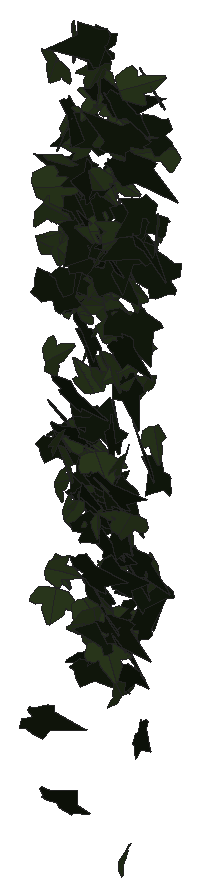
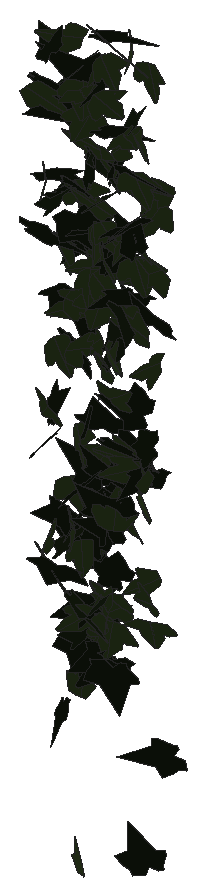
# SketchUp Ruby script. Lengths in inches.
U = 1.inch
M = Sketchup.active_model
def pt(a) = Geom::Point3d.new(a.map { |v| v * U })
def face(e, loops, mat)
  f = e.add_face(loops[0].map { |a| pt(a) })
  loops[1..].each { |l| e.add_face(l.map { |a| pt(a) }).erase! }
  f.material = f.back_material = mat if mat
  f
end
# faces: each face lists its corners as indices into pts; further lists are holes
def faces(e, pts, list, mat = nil) = list.each { |f| face(e, (f[0].is_a?(Array) ? f : [f]).map { |l| l.map { |i| pts[i] } }, mat) }
# xy, xz, yz: faces in a plane at the given z, y or x. An outline is a flat list of corners, or four numbers for a rectangle; further outlines are holes
def ring(l) = l.size == 4 ? [[l[0], l[1]], [l[2], l[1]], [l[2], l[3]], [l[0], l[3]]] : l.each_slice(2).to_a
def flat(e, list, mat, &to3) = list.each { |f| face(e, (f[0].is_a?(Array) ? f : [f]).map { |l| ring(l).map { |u, v| to3.(u, v) } }, mat) }
def xy(e, z, list, mat = nil) = flat(e, list, mat) { |x, y| [x, y, z] }
def xz(e, y, list, mat = nil) = flat(e, list, mat) { |x, z| [x, y, z] }
def yz(e, x, list, mat = nil) = flat(e, list, mat) { |y, z| [x, y, z] }
def lines(e, pts, list) = list.each { |a, b| e.add_line(pt(pts[a]), pt(pts[b])) }
# prism: a flat outline (further loops are holes) pulled along v
def prism(e, loops, v, mat = nil)
  f = face(e, loops, mat); d = Geom::Vector3d.new(v.map { |x| x * U })
  f.pushpull(f.normal.samedirection?(d) ? d.length : -d.length)
end
def box(e, o, s, mat = nil) = prism(e, [[o, [o[0] + s[0], o[1], o[2]], [o[0] + s[0], o[1] + s[1], o[2]], [o[0], o[1] + s[1], o[2]]]], [0, 0, s[2]], mat)
def at(x, y, z, deg = 0) = Geom::Transformation.translation(pt([x, y, z])) * Geom::Transformation.rotation(ORIGIN, Z_AXIS, deg.degrees)
def axes(o, x, y, z) = Geom::Transformation.new([*x, 0, *y, 0, *z, 0, *pt(o).to_a, 1])
def part(name) = M.definitions.add(name)
# library, detail: a bought-in or finely detailed component or shape, given as its bounding box
def library(name, o, s) = part(name).tap { |d| box(d.entities, o, s) }
def detail(e, o, s) = box(e.add_group.entities, o, s)
def put(e, d, t, mat = nil) = e.add_instance(d, t).tap { |i| i.material = mat if mat }
def group(e, t, mat = nil) = e.add_group.tap { |g| g.transformation = t; g.material = mat if mat }.entities
root = M.entities
M.materials.add("1026 AP 7946 SUNNY SIDE UP").color = [254, 231, 186]
M.materials.add("efeu1").color = [18, 25, 13]
M.materials.add("efeu2").color = [43, 57, 29]
c1 = part("ivyleaf_10")
p = [[0,0.5,-0.03],[-0.0625,2.02,-0.43],[-0.19,2.01,-0.46],[-0.54,1.05,-0.29],[-0.52,0.625,-0.18],[-0.83,0.76,-0.28],
  [-1.16,0.64,-0.33],[-1.15,0.33,-0.24],[-0.77,-0.39,0.02],[-0.3,-0.51,0.16],[0.04,-0.48,0.23],[-0.02,2.01,-0.4375],
  [-0.06,2.01,-0.43],[0.04,-0.49,0.23],[0.67,-0.49,0.14],[1.38,0.36,-0.2],[1.375,0.51,-0.24],[0.81,0.65,-0.19],
  [0.62,0.59,-0.15],[0.6,1.09,-0.28],[0.5,1.23,-0.31]]
faces(c1.entities,p,[[0,1,2,3,4,5,6,7,8,9,10],[11,12,0,13,14,15,16,17,18,19,20]],"efeu2")
c2 = part("ivyleaf_9")
p = [[1.54,2.16,1.25],[1.36,2.04,1.19],[-0.21,0.99,0.68],[-0.71,1.11,0.82],[-0.85,0.86,0.67],[-0.8,0.17,0.21],
  [-0.9,-0.01,0.1],[-0.67,-0.16,-0.02],[-0.08,-0.08,-0.05],[-0.03,-0.6,-0.4],[0.65,-0.88,-0.66],[0.83,-0.6,-0.49],
  [1.29,-0.42,-0.43],[1.8125,-0.07,-0.26],[1.21,0.44,0.15]]
faces(c2.entities,p,[[0,1,2,3,4,5,6,7,8,9,10,11,12,13,14]],"efeu1")
put(root,c1,axes([114.66,211.24,255.74],[-0.17007,-0.25209,-0.06808],[0.06713,0.05188,-0.28166],[0.40367,-0.11483,0.01816]),"1026 AP 7946 SUNNY SIDE UP")
put(root,c2,axes([114.43,211.45,264.72],[-0.03264,-0.0088,0.26998],[-0.17282,-0.23845,-0.01861],[0.37443,-0.11082,0.01495]),"1026 AP 7946 SUNNY SIDE UP")
put(root,c1,axes([115.3,211.32,264.08],[-0.30301,-0.12678,0.13717],[-0.15655,-0.09143,-0.23738],[0.244,-0.21609,0.01804]),"1026 AP 7946 SUNNY SIDE UP")
put(root,c1,axes([114.875,211.3,255],[0.39379,0.04754,0.12039],[0.18826,-0.00959,-0.26097],[-0.06127,0.27608,-0.02813]),"1026 AP 7946 SUNNY SIDE UP")
put(root,c1,axes([113.82,211.09,256.41],[0.04108,0.08662,0.235],[0.07694,0.22239,-0.09167],[-0.37514,0.0551,0.00693]),"1026 AP 7946 SUNNY SIDE UP")
put(root,c2,axes([114.28,211.5,263.51],[-0.16249,-0.21094,0.17183],[-0.07271,-0.16337,-0.2416],[0.41773,-0.11049,0.02478]),"1026 AP 7946 SUNNY SIDE UP")
put(root,c2,axes([115.59,211.3,257.2],[0.02088,-0.02394,-0.25705],[0.3777,0.07217,0.00646],[0.11192,-0.23908,0.02615]),"1026 AP 7946 SUNNY SIDE UP")
put(root,c2,axes([115.05,211.33,256.57],[0.04614,0.00383,0.26116],[0.28307,-0.17999,-0.01972],[0.28067,0.18089,-0.02304]),"1026 AP 7946 SUNNY SIDE UP")
put(root,c2,axes([115.49,211.22,265.66],[-0.01709,-0.02402,-0.30405],[0.35249,0.19209,-0.02349],[0.30389,-0.22416,0.01015]),"1026 AP 7946 SUNNY SIDE UP")
put(root,c2,axes([115.65,211.44,263.92],[-0.30341,-0.11682,0.11722],[-0.13955,-0.07389,-0.23227],[0.216,-0.21183,0.0146]),"1026 AP 7946 SUNNY SIDE UP")
put(root,c1,axes([113.54,211.17,264.51],[0.12534,-0.00768,-0.2999],[0.42709,0.11067,0.07427],[0.16492,-0.28076,0.03558]),"1026 AP 7946 SUNNY SIDE UP")
put(root,c1,axes([113.61,211.15,264.12],[-0.1046,-0.20587,-0.24089],[0.18057,0.20479,-0.21931],[0.4539,-0.12891,0.03173]),"1026 AP 7946 SUNNY SIDE UP")
put(root,c2,axes([114.8,211.375,258.32],[0.04947,-0.07557,0.27589],[0.34471,-0.15995,-0.07385],[0.27054,0.21762,0.04365]),"1026 AP 7946 SUNNY SIDE UP")
put(root,c1,axes([114.51,211.43,257.81],[0.22659,-0.07934,0.20756],[0.24435,-0.13141,-0.16821],[0.23805,0.21041,-0.0249]),"1026 AP 7946 SUNNY SIDE UP")
put(root,c2,axes([115.31,211.41,260.83],[-0.18396,-0.02952,-0.27245],[0.41815,-0.01085,-0.12008],[0.0031,-0.28883,0.03065]),"1026 AP 7946 SUNNY SIDE UP")
put(root,c2,axes([114.97,211.49,255.23],[-0.12645,-0.02112,0.26836],[-0.28963,-0.18894,-0.07543],[0.29179,-0.19669,0.04142]),"1026 AP 7946 SUNNY SIDE UP")
put(root,c2,axes([114.96,211.24,263.16],[0.11119,-0.17412,-0.20533],[-0.01889,0.20299,-0.18682],[0.41455,0.05595,0.04656]),"1026 AP 7946 SUNNY SIDE UP")
put(root,c1,axes([114.98,211.4,265.1],[-0.07258,-0.05386,-0.264],[0.34796,-0.14661,-0.01019],[-0.21927,-0.21483,0.07122]),"1026 AP 7946 SUNNY SIDE UP")
put(root,c1,axes([114.59,211.4,264.96],[-0.22027,0.03601,-0.22286],[0.26472,-0.14719,-0.13829],[-0.22147,-0.21176,0.05635]),"1026 AP 7946 SUNNY SIDE UP")
put(root,c2,axes([115.13,211.4,261.6],[0.0724,-0.05469,-0.27668],[0.42883,0.03311,0.04146],[0.0379,-0.27017,0.05943]),"1026 AP 7946 SUNNY SIDE UP")
put(root,c2,axes([114.66,211.5,263.34],[0.09706,-0.13204,0.269],[0.13776,-0.24708,-0.15107],[0.44008,0.10646,-0.01204]),"1026 AP 7946 SUNNY SIDE UP")
put(root,c2,axes([116,211.25,259.24],[0.00962,-0.17645,0.2395],[-0.01877,0.23319,0.18324],[-0.4598,-0.01321,-0.00247]),"1026 AP 7946 SUNNY SIDE UP")
put(root,c1,axes([115.4,211.36,257.95],[-0.33522,-0.14331,0.08976],[-0.09251,-0.06946,-0.26394],[0.24768,-0.21991,0.02291]),"1026 AP 7946 SUNNY SIDE UP")
put(root,c1,axes([113.6,211.36,255.67],[0.38787,0.0925,-0.01096],[-0.00313,-0.02634,-0.27043],[-0.14647,0.24552,-0.02323]),"1026 AP 7946 SUNNY SIDE UP")
put(root,c2,axes([114.35,211.38,256.41],[0.08918,-0.01835,0.26004],[0.30281,-0.16487,-0.05787],[0.25845,0.1995,-0.02193]),"1026 AP 7946 SUNNY SIDE UP")
put(root,c1,axes([114.86,211.39,261.15],[-0.24924,0.15249,-0.16603],[0.15304,-0.13138,-0.22624],[-0.31462,-0.18471,0.02148]),"1026 AP 7946 SUNNY SIDE UP")
put(root,c2,axes([113.28,211.19,253.03],[0.1264,0.03867,-0.24017],[0.12708,0.22714,0.06879],[0.34954,-0.09656,0.06184]),"1026 AP 7946 SUNNY SIDE UP")
put(root,c2,axes([114.92,211.29,255.56],[-0.03216,-0.04064,-0.27817],[0.30762,0.18639,-0.04311],[0.29902,-0.19612,0.01444]),"1026 AP 7946 SUNNY SIDE UP")
put(root,c2,axes([115.7,211.31,255.73],[-0.09753,0.22615,0.16908],[0.07272,-0.15616,0.24065],[0.43212,0.07732,-0.00234]),"1026 AP 7946 SUNNY SIDE UP")
put(root,c1,axes([113.8,211.38,258.8],[-0.21862,0.17295,-0.11784],[0.09605,-0.09868,-0.22881],[-0.31247,-0.15134,0.01212]),"1026 AP 7946 SUNNY SIDE UP")
put(root,c1,axes([114.41,211.35,255.73],[0.29749,0.06497,0.17027],[0.26175,0.01771,-0.20383],[-0.09571,0.25035,-0.0282]),"1026 AP 7946 SUNNY SIDE UP")
put(root,c1,axes([113.69,211.13,260.9],[0.04669,-0.00574,-0.30414],[0.15125,0.28068,0.00598],[0.43892,-0.09611,0.03029]),"1026 AP 7946 SUNNY SIDE UP")
put(root,c2,axes([114.72,211.49,256.97],[0.07288,-0.04471,0.28318],[0.22679,-0.23482,-0.06571],[0.37505,0.15068,-0.01529]),"1026 AP 7946 SUNNY SIDE UP")
put(root,c1,axes([114.55,211.36,255.27],[-0.42453,-0.06949,-0.01035],[0.02571,-0.02499,-0.28587],[0.10728,-0.269,0.02753]),"1026 AP 7946 SUNNY SIDE UP")
put(root,c2,axes([115.36,211.39,265.92],[0.00099,0.0417,0.27274],[-0.41206,0.0545,-0.00789],[-0.0866,-0.25884,0.04066]),"1026 AP 7946 SUNNY SIDE UP")
put(root,c2,axes([114.54,211.4375,257.76],[0.30374,-0.14164,0.10657],[-0.1091,0.08092,0.24617],[-0.2541,-0.20404,0.02169]),"1026 AP 7946 SUNNY SIDE UP")
put(root,c1,axes([113.63,211.5,258.05],[0.08777,-0.1533,-0.2045],[0.15271,-0.17333,0.16575],[-0.36243,-0.11015,0.02031]),"1026 AP 7946 SUNNY SIDE UP")
put(root,c2,axes([114.36,211.44,257.76],[-0.00977,-0.02193,0.26649],[0.28374,-0.18656,-0.01292],[0.29374,0.17948,0.02134]),"1026 AP 7946 SUNNY SIDE UP")
put(root,c2,axes([115.18,211.33,257.51],[0.17287,-0.16507,-0.15645],[-0.15698,0.11428,-0.20301],[0.31472,0.14767,-0.01532]),"1026 AP 7946 SUNNY SIDE UP")
put(root,c1,axes([114.56,211.48,255.8],[-0.13203,0.02969,0.24357],[0.33412,-0.10372,0.09062],[0.16897,0.22828,0.01113]),"1026 AP 7946 SUNNY SIDE UP")
put(root,c2,axes([114.22,211.59,261.51],[0.04531,-0.20769,0.19512],[0.03591,-0.18923,-0.2171],[0.44178,0.03668,-0.00237]),"1026 AP 7946 SUNNY SIDE UP")
put(root,c1,axes([113.72,211.43,259.14],[0.05475,-0.24728,0.00725],[-0.00329,-0.00881,-0.25728],[0.38903,0.03472,-0.00319]),"1026 AP 7946 SUNNY SIDE UP")
put(root,c2,axes([114.27,211.62,261.06],[-0.03174,-0.12777,0.26578],[0.03799,-0.25919,-0.13144],[0.45212,0.01281,0.0297]),"1026 AP 7946 SUNNY SIDE UP")
put(root,c1,axes([114.67,211.39,263.85],[0.20477,-0.05823,-0.22915],[0.35388,-0.01823,0.14076],[-0.07154,-0.25682,0.04038]),"1026 AP 7946 SUNNY SIDE UP")
put(root,c1,axes([113.96,211.41,257.5],[0.32931,-0.17306,-0.04965],[0.08071,-0.01173,0.27878],[-0.27028,-0.21436,0.02275]),"1026 AP 7946 SUNNY SIDE UP")
put(root,c1,axes([114.62,211.4,258.91],[0.33119,0.14616,0.07968],[0.11985,0.02385,-0.26292],[-0.23008,0.22282,-0.02225]),"1026 AP 7946 SUNNY SIDE UP")
put(root,c1,axes([113.68,211.37,267.09],[-0.34648,0.10045,0.1055],[-0.17571,-0.00413,-0.24493],[-0.14042,-0.24271,0.04617]),"1026 AP 7946 SUNNY SIDE UP")
put(root,c2,axes([115.26,211.36,254.75],[0.31164,0.03666,-0.16069],[-0.23369,-0.05154,-0.20705],[-0.09501,0.24702,-0.01781]),"1026 AP 7946 SUNNY SIDE UP")
put(root,c2,axes([113.73,211.51,260.06],[0.2403,-0.11574,0.21856],[0.23253,-0.15472,-0.197],[0.3017,0.21144,-0.02225]),"1026 AP 7946 SUNNY SIDE UP")
put(root,c1,axes([113.52,211.51,256.24],[0.16121,-0.00611,0.21576],[0.3107,-0.07483,-0.10232],[0.10972,0.22088,-0.02726]),"1026 AP 7946 SUNNY SIDE UP")
put(root,c2,axes([113.93,211.6875,265.85],[-0.02854,-0.19514,0.25533],[-0.02292,-0.24858,-0.20329],[0.49685,-0.02267,0.00529]),"1026 AP 7946 SUNNY SIDE UP")
put(root,c2,axes([114.56,211.32,254.6],[-0.00266,-0.10371,-0.2671],[0.01774,0.25845,-0.10531],[0.43787,-0.0111,0.00265]),"1026 AP 7946 SUNNY SIDE UP")
put(root,c1,axes([115.06,211.59,253.98],[-0.08601,-0.20779,-0.16962],[-0.04609,-0.16113,0.22017],[-0.41316,0.06123,0.01075]),"1026 AP 7946 SUNNY SIDE UP")
put(root,c2,axes([114.72,211.47,262.72],[0.13518,-0.1909,0.13804],[-0.02992,0.13773,0.2138],[-0.36649,-0.08165,0.03346]),"1026 AP 7946 SUNNY SIDE UP")
put(root,c1,axes([115.13,211.67,260.94],[-0.0853,-0.03267,0.29358],[0.02072,-0.29018,-0.03337],[0.45084,0.00716,0.05708]),"1026 AP 7946 SUNNY SIDE UP")
put(root,c1,axes([114.13,211.625,265.4],[-0.04069,0.09275,0.24744],[0.02887,-0.23959,0.09617],[0.40305,0.02652,0.01809]),"1026 AP 7946 SUNNY SIDE UP")
put(root,c2,axes([115.42,211.54,264.3125],[-0.38926,0.02006,-0.04618],[0.06741,-0.02532,-0.25506],[-0.03801,-0.25033,0.02061]),"1026 AP 7946 SUNNY SIDE UP")
put(root,c2,axes([114.38,211.31,257.33],[0.053,0.04424,0.26084],[0.37301,0.09229,-0.04866],[-0.15456,0.2379,-0.02798]),"1026 AP 7946 SUNNY SIDE UP")
put(root,c2,axes([114.53,211.41,258.38],[-0.20288,0.10014,0.21062],[0.27908,-0.10187,0.16667],[0.22288,0.21871,-0.01698]),"1026 AP 7946 SUNNY SIDE UP")
put(root,c2,axes([114.48,211.57,256.03],[0.15726,-0.25847,0.02263],[0.0048,-0.02393,-0.2856],[0.40806,0.0999,-0.00536]),"1026 AP 7946 SUNNY SIDE UP")
put(root,c1,axes([113.76,211.5625,265.73],[0.19013,-0.21589,0.08202],[0.04409,-0.07684,-0.25504],[0.35979,0.1235,-0.01209]),"1026 AP 7946 SUNNY SIDE UP")
put(root,c1,axes([115.32,211.59,262.68],[-0.13872,0.07861,0.27248],[0.36566,-0.12742,0.11838],[0.23228,0.24753,-0.02362]),"1026 AP 7946 SUNNY SIDE UP")
put(root,c1,axes([115.17,211.47,259.15],[0.04188,-0.28273,-0.06084],[-0.00235,0.05756,-0.2922],[0.45365,0.0264,0.0041]),"1026 AP 7946 SUNNY SIDE UP")
put(root,c2,axes([114.97,211.57,255.19],[0.22849,-0.21422,0.05526],[0.02806,-0.05407,-0.26652],[0.34657,0.14561,-0.01486]),"1026 AP 7946 SUNNY SIDE UP")
put(root,c2,axes([114.68,211.42,259.44],[-0.32119,-0.00531,0.14945],[0.22806,-0.01912,0.20952],[0.01063,0.24983,0.02068]),"1026 AP 7946 SUNNY SIDE UP")
put(root,c2,axes([114.54,211.62,267.64],[-0.33393,-0.00971,0.16324],[-0.2327,-0.0839,-0.21005],[0.09058,-0.25137,0.06217]),"1026 AP 7946 SUNNY SIDE UP")
put(root,c1,axes([114.43,211.61,260.74],[0.05075,-0.08601,-0.23648],[0.23756,-0.17473,0.0885],[-0.30262,-0.15159,0.02982]),"1026 AP 7946 SUNNY SIDE UP")
put(root,c2,axes([115.51,211.59,263.96],[0.20555,-0.25103,0.03547],[0.01146,-0.0366,-0.29159],[0.39856,0.13051,-0.00991]),"1026 AP 7946 SUNNY SIDE UP")
put(root,c1,axes([115.15,211.67,261.95],[-0.05558,-0.12647,0.22673],[-0.05695,-0.21815,-0.13597],[0.39603,-0.04912,0.01227]),"1026 AP 7946 SUNNY SIDE UP")
put(root,c2,axes([113.78,211.5625,259.05],[0.37981,-0.02151,-0.02187],[0.03629,0.02235,0.24871],[-0.03048,-0.24144,0.02354]),"1026 AP 7946 SUNNY SIDE UP")
put(root,c2,axes([114.18,211.46,264.85],[-0.19437,0.13254,0.19459],[-0.29028,0.07039,-0.17564],[-0.21604,-0.21382,0.06093]),"1026 AP 7946 SUNNY SIDE UP")
put(root,c1,axes([115.58,211.58,260.85],[-0.11909,-0.27542,0.06823],[-0.01917,-0.06694,-0.2946],[0.44559,-0.07649,0.00556]),"1026 AP 7946 SUNNY SIDE UP")
put(root,c2,axes([114.91,211.62,263.47],[-0.10304,-0.2649,-0.05673],[0.02722,0.05089,-0.28078],[0.42408,-0.06763,0.00424]),"1026 AP 7946 SUNNY SIDE UP")
put(root,c1,axes([114.51,211.58,263.62],[-0.27553,-0.13701,0.11319],[-0.11756,-0.08345,-0.22892],[0.25073,-0.1897,0.01705]),"1026 AP 7946 SUNNY SIDE UP")
put(root,c2,axes([115.06,211.51,266.81],[0.22169,-0.22399,-0.11841],[-0.05999,0.10974,-0.27089],[0.39038,0.14407,0.02561]),"1026 AP 7946 SUNNY SIDE UP")
put(root,c1,axes([115.77,211.66,256.74],[-0.10353,0.13953,0.22415],[0.15244,-0.19393,0.15779],[0.37563,0.11716,-0.00225]),"1026 AP 7946 SUNNY SIDE UP")
put(root,c2,axes([114.41,211.68,265.74],[-0.3294,-0.08627,0.13607],[-0.16654,-0.0869,-0.23118],[0.18472,-0.23219,0.03423]),"1026 AP 7946 SUNNY SIDE UP")
put(root,c2,axes([115.13,211.57,263.66],[-0.00973,0.20677,-0.223],[-0.03129,-0.21748,-0.21355],[-0.47099,0.01018,0.01879]),"1026 AP 7946 SUNNY SIDE UP")
put(root,c2,axes([115.71,211.7,264.42],[-0.32129,-0.13757,0.1002],[-0.10281,-0.07748,-0.25282],[0.24493,-0.21298,0.02532]),"1026 AP 7946 SUNNY SIDE UP")
put(root,c1,axes([113.83,211.55,264.87],[-0.36323,-0.04128,0.10677],[-0.14616,-0.06152,-0.2385],[0.09763,-0.2457,0.0402]),"1026 AP 7946 SUNNY SIDE UP")
put(root,c1,axes([115.38,211.36,267.18],[0.12226,0.03109,-0.29225],[0.3264,0.19587,0.08182],[0.30834,-0.21967,0.02927]),"1026 AP 7946 SUNNY SIDE UP")
put(root,c2,axes([114.67,211.34,264.73],[-0.2767,0.21118,-0.08365],[-0.06078,0.07483,0.28305],[0.35122,0.17932,-0.01692]),"1026 AP 7946 SUNNY SIDE UP")
put(root,c2,axes([115.16,211.68,257.05],[0.15116,-0.28344,0.06843],[0.02159,-0.06716,-0.30861],[0.45784,0.09675,-0.00804]),"1026 AP 7946 SUNNY SIDE UP")
put(root,c2,axes([113.53,211.45,261.98],[-0.28326,0.18516,0.18087],[0.22182,-0.10528,0.26447],[0.33298,0.22765,-0.02231]),"1026 AP 7946 SUNNY SIDE UP")
put(root,c1,axes([114.97,211.48,261.9],[-0.26387,-0.0846,-0.26562],[0.40009,0.05468,-0.18913],[0.14621,-0.30233,0.03816]),"1026 AP 7946 SUNNY SIDE UP")
put(root,c2,axes([115,211.4375,259.34],[-0.05752,-0.13647,0.24371],[0.11734,0.22541,0.14669],[-0.41419,0.08281,0.00772]),"1026 AP 7946 SUNNY SIDE UP")
put(root,c2,axes([115.27,211.58,262.11],[-0.12016,-0.22665,-0.17988],[0.09067,0.16346,-0.24545],[0.4394,-0.09571,0.00145]),"1026 AP 7946 SUNNY SIDE UP")
put(root,c1,axes([114.6,211.66,266.98],[-0.00117,0.20336,-0.17163],[-0.05023,-0.16658,-0.20887],[-0.41146,0.01975,0.02599]),"1026 AP 7946 SUNNY SIDE UP")
put(root,c1,axes([115.8,211.71,264.24],[-0.06976,0.1297,-0.23697],[0.06035,-0.22835,-0.14116],[-0.41183,-0.05543,0.01946]),"1026 AP 7946 SUNNY SIDE UP")
put(root,c2,axes([114.79,211.54,266.54],[0.01605,-0.01632,0.32334],[0.4715,-0.09385,-0.01562],[0.14849,0.29977,0.01464]),"1026 AP 7946 SUNNY SIDE UP")
put(root,c1,axes([113.95,211.58,261.91],[-0.23222,0.02323,0.23306],[0.35732,0.02044,0.15087],[-0.00709,0.26929,-0.02996]),"1026 AP 7946 SUNNY SIDE UP")
put(root,c1,axes([114.93,211.55,265.78],[-0.3757,-0.08453,-0.08112],[0.12979,0.00008,-0.25969],[0.12635,-0.25142,0.02556]),"1026 AP 7946 SUNNY SIDE UP")
put(root,c2,axes([114.2,211.55,263.11],[0.00623,-0.19021,-0.16302],[-0.01234,0.15701,-0.19505],[0.38778,0.00805,-0.00359]),"1026 AP 7946 SUNNY SIDE UP")
put(root,c1,axes([113.41,211.57,263.12],[-0.33087,-0.00171,-0.20168],[0.3042,-0.0458,-0.21409],[-0.04711,-0.28373,0.03406]),"1026 AP 7946 SUNNY SIDE UP")
put(root,c1,axes([114.23,211.68,257.75],[-0.20254,-0.2531,-0.1013],[-0.0817,-0.08222,0.29195],[-0.41823,0.13864,-0.00798]),"1026 AP 7946 SUNNY SIDE UP")
put(root,c2,axes([115.57,211.46,253.38],[0.08727,-0.08953,-0.24019],[-0.26492,0.16219,-0.10475],[0.28888,0.17578,-0.02351]),"1026 AP 7946 SUNNY SIDE UP")
put(root,c2,axes([114.7,211.53,266.68],[0.34275,-0.09494,-0.11264],[-0.1687,0.02536,-0.2441],[0.15196,0.2423,-0.01694]),"1026 AP 7946 SUNNY SIDE UP")
put(root,c1,axes([114.98,211.69,250.35],[0.08828,-0.18817,-0.15191],[0.07578,-0.13833,0.20141],[-0.36713,-0.0738,0.00505]),"1026 AP 7946 SUNNY SIDE UP")
put(root,c1,axes([113.78,211.75,267.625],[-0.05443,0.13762,-0.26838],[0.08631,-0.2555,-0.14762],[-0.45628,-0.06475,0.00409]),"1026 AP 7946 SUNNY SIDE UP")
put(root,c2,axes([113.42,211.61,259.52],[0.32069,-0.14904,0.03234],[0.02365,-0.0339,-0.25974],[0.2386,0.20368,-0.01771]),"1026 AP 7946 SUNNY SIDE UP")
put(root,c2,axes([114.45,211.78,264.3],[-0.05739,-0.24369,0.11322],[0.01193,-0.11321,-0.25349],[0.42107,-0.03001,0.02261]),"1026 AP 7946 SUNNY SIDE UP")
put(root,c1,axes([113.61,211.7,263.67],[0.26768,-0.13845,0.11008],[0.10767,-0.08564,-0.22553],[0.25387,0.1823,-0.02042]),"1026 AP 7946 SUNNY SIDE UP")
put(root,c1,axes([115.01,211.61,256.89],[-0.18088,-0.22644,-0.01459],[0.02704,0.00569,-0.26129],[0.3556,-0.11561,0.01245]),"1026 AP 7946 SUNNY SIDE UP")
put(root,c2,axes([113.51,211.5,258.93],[0.03453,-0.11774,-0.2365],[-0.02651,0.22858,-0.12146],[0.40388,0.02507,0.01225]),"1026 AP 7946 SUNNY SIDE UP")
put(root,c1,axes([114.09,211.42,263.5],[0.01483,0.15866,0.22379],[-0.08145,0.21347,-0.15771],[-0.4139,-0.03632,0.03905]),"1026 AP 7946 SUNNY SIDE UP")
put(root,c2,axes([115.98,211.64,266.23],[-0.36015,0.06891,0.09272],[-0.14263,0.00879,-0.24576],[-0.10608,-0.24579,0.01565]),"1026 AP 7946 SUNNY SIDE UP")
put(root,c1,axes([113.72,211.65,263.18],[-0.2925,-0.19711,0.06224],[-0.04119,-0.05963,-0.27869],[0.32207,-0.18664,0.02089]),"1026 AP 7946 SUNNY SIDE UP")
put(root,c2,axes([114.36,211.54,254.58],[0.1362,0.22546,-0.09785],[-0.04523,-0.09204,-0.24929],[-0.38282,0.09109,-0.00536]),"1026 AP 7946 SUNNY SIDE UP")
put(root,c2,axes([114.65,211.41,254.72],[-0.02008,0.09683,-0.2391],[-0.08431,0.22656,0.10151],[0.38716,0.05436,0.0097]),"1026 AP 7946 SUNNY SIDE UP")
put(root,c2,axes([115.1875,211.6,255.76],[-0.27125,0.19469,-0.03868],[0.02,-0.04026,-0.26764],[-0.31146,-0.17214,0.0165]),"1026 AP 7946 SUNNY SIDE UP")
put(root,c1,axes([116.05,211.64,265.95],[0.23365,0.01355,-0.2306],[-0.35272,0.01068,-0.15263],[0.00224,0.26852,0.01929]),"1026 AP 7946 SUNNY SIDE UP")
put(root,c1,axes([114.73,211.5,263.46],[-0.00989,-0.22857,-0.19857],[-0.00613,0.19155,-0.23433],[0.46879,-0.00232,-0.00725]),"1026 AP 7946 SUNNY SIDE UP")
put(root,c1,axes([113.89,211.625,259.15],[0.0977,0.04531,0.28171],[0.4282,0.04087,-0.07055],[-0.07912,0.27718,-0.03395]),"1026 AP 7946 SUNNY SIDE UP")
put(root,c2,axes([114.88,211.67,258.31],[0.15267,-0.2755,-0.10374],[-0.05263,0.09331,-0.30038],[0.45737,0.1027,0.00006]),"1026 AP 7946 SUNNY SIDE UP")
put(root,c1,axes([114.41,211.7,267.12],[-0.11837,-0.24992,0.06226],[-0.02328,-0.06013,-0.26923],[0.40417,-0.07666,0.00272]),"1026 AP 7946 SUNNY SIDE UP")
put(root,c1,axes([114.75,211.46,262.75],[-0.00446,0.00574,0.25674],[0.1038,0.24031,-0.00352],[-0.37792,0.06594,-0.004]),"1026 AP 7946 SUNNY SIDE UP")
put(root,c2,axes([115.56,211.82,267.06],[0.02668,-0.13006,0.23525],[0.09507,-0.22152,-0.13547],[0.40318,0.06084,0.01637]),"1026 AP 7946 SUNNY SIDE UP")
put(root,c1,axes([114.5,211.75,262.65],[-0.06489,-0.23368,0.12018],[-0.02796,-0.11666,-0.24513],[0.41066,-0.04487,0.0023]),"1026 AP 7946 SUNNY SIDE UP")
put(root,c1,axes([114.33,211.79,263.11],[0.22426,-0.10012,0.24371],[0.28699,-0.15183,-0.18002],[0.28541,0.23135,-0.01048]),"1026 AP 7946 SUNNY SIDE UP")
put(root,c2,axes([114.67,211.83,264.7],[0.00226,-0.03883,0.26667],[0.0031,-0.25907,-0.04153],[0.41191,0.00216,-0.00115]),"1026 AP 7946 SUNNY SIDE UP")
put(root,c2,axes([114.61,211.61,267.6],[-0.3286,0.17909,0.10321],[-0.15033,0.03993,-0.2816],[-0.28463,-0.22784,0.02958]),"1026 AP 7946 SUNNY SIDE UP")
put(root,c1,axes([114.86,211.59,255.5625],[-0.24347,-0.11475,-0.20034],[0.29169,0.06843,-0.19401],[0.20087,-0.23845,0.0389]),"1026 AP 7946 SUNNY SIDE UP")
put(root,c1,axes([113.52,211.73,261.87],[-0.02424,0.03045,0.28065],[0.42229,-0.0521,0.02137],[0.08495,0.26766,-0.02612]),"1026 AP 7946 SUNNY SIDE UP")
put(root,c1,axes([114.57,211.66,262.13],[-0.40803,-0.06378,-0.03767],[0.06437,-0.01553,-0.27421],[0.09568,-0.26155,0.02384]),"1026 AP 7946 SUNNY SIDE UP")
put(root,c1,axes([114.91,211.74,266.38],[0.25876,0.18042,-0.10446],[-0.08524,-0.08879,-0.25139],[-0.31489,0.1723,-0.01778]),"1026 AP 7946 SUNNY SIDE UP")
put(root,c2,axes([113.63,211.82,263.64],[0.02067,-0.04639,0.27583],[0.16777,-0.24593,-0.05068],[0.3934,0.10732,0.00712]),"1026 AP 7946 SUNNY SIDE UP")
put(root,c1,axes([113.73,211.64,258.97],[-0.25069,-0.04035,-0.23737],[0.36432,0.00902,-0.16691],[0.04788,-0.27986,0.02717]),"1026 AP 7946 SUNNY SIDE UP")
put(root,c1,axes([114.95,211.68,266.4],[-0.43465,-0.05307,0.02078],[-0.02346,-0.03036,-0.28882],[0.08631,-0.27551,0.02613]),"1026 AP 7946 SUNNY SIDE UP")
put(root,c1,axes([114.2,211.78,261.26],[0.14733,-0.22417,0.09435],[0.04876,-0.08766,-0.25076],[0.3784,0.09857,-0.00443]),"1026 AP 7946 SUNNY SIDE UP")
put(root,c1,axes([114.38,211.85,266.44],[-0.15904,-0.17702,0.19859],[-0.02435,-0.20328,-0.20082],[0.41197,-0.08035,0.0648]),"1026 AP 7946 SUNNY SIDE UP")
put(root,c2,axes([115.47,211.77,256.43],[-0.25235,-0.15446,-0.17867],[0.24982,0.07932,-0.22491],[0.26495,-0.2219,0.04188]),"1026 AP 7946 SUNNY SIDE UP")
put(root,c1,axes([114.77,211.67,262.59],[-0.14922,-0.2407,-0.04871],[0.04704,0.03749,-0.26594],[0.38242,-0.09853,0.01371]),"1026 AP 7946 SUNNY SIDE UP")
put(root,c1,axes([113.89,211.78,265.86],[0.15229,0.18956,-0.15057],[-0.07262,-0.14108,-0.21925],[-0.37036,0.10561,-0.01892]),"1026 AP 7946 SUNNY SIDE UP")
put(root,c1,axes([115.62,211.8,259.65],[0.27783,-0.06804,0.18797],[0.24621,-0.0977,-0.1939],[0.18299,0.23475,-0.02449]),"1026 AP 7946 SUNNY SIDE UP")
put(root,c2,axes([115.74,211.91,258.83],[-0.08095,-0.17186,0.19271],[-0.07185,-0.1825,-0.18579],[0.39407,-0.06858,0.00571]),"1026 AP 7946 SUNNY SIDE UP")
put(root,c2,axes([116.04,211.71,263.14],[-0.309,0.09315,0.19299],[-0.28951,0.04355,-0.22165],[-0.15466,-0.26762,0.02931]),"1026 AP 7946 SUNNY SIDE UP")
put(root,c1,axes([114.25,211.67,260.27],[0.29123,0.01856,0.15439],[-0.23713,0.01428,0.1904],[0.0085,-0.23775,0.02208]),"1026 AP 7946 SUNNY SIDE UP")
put(root,c2,axes([113.76,211.8,264.1],[0.08643,-0.26169,-0.02455],[-0.01149,0.02129,-0.27534],[0.41283,0.05538,-0.00253]),"1026 AP 7946 SUNNY SIDE UP")
put(root,c2,axes([113.85,211.84,264.03],[-0.06433,-0.29061,-0.01963],[0.01615,0.01613,-0.30213],[0.45748,-0.04143,0.00791]),"1026 AP 7946 SUNNY SIDE UP")
put(root,c2,axes([113.38,211.76,251],[0.38556,0.00713,-0.00574],[0.00733,0.03114,0.25088],[0.01224,-0.24329,0.03049]),"1026 AP 7946 SUNNY SIDE UP")
put(root,c2,axes([114.24,211.78,259.39],[-0.38791,0.03864,0.07144],[-0.11277,-0.01307,-0.25622],[-0.05283,-0.25587,0.02234]),"1026 AP 7946 SUNNY SIDE UP")
put(root,c2,axes([113.82,211.67,262.56],[0.06828,-0.16252,-0.22164],[0.1371,0.21378,-0.14762],[0.39995,-0.04554,0.08844]),"1026 AP 7946 SUNNY SIDE UP")
put(root,c1,axes([115.01,211.89,257.4],[-0.08696,0.10555,-0.27157],[0.1125,-0.25534,-0.12201],[-0.43299,-0.08754,0.02284]),"1026 AP 7946 SUNNY SIDE UP")
put(root,c2,axes([114.3,211.62,257.86],[-0.19198,0.02444,0.25831],[0.39583,0.01765,0.12468],[-0.00825,0.2782,-0.02896]),"1026 AP 7946 SUNNY SIDE UP")
put(root,c2,axes([114.06,211.52,262.04],[0.00789,0.2239,0.16265],[-0.0075,0.15669,-0.2297],[-0.42958,0.00138,0.007]),"1026 AP 7946 SUNNY SIDE UP")
